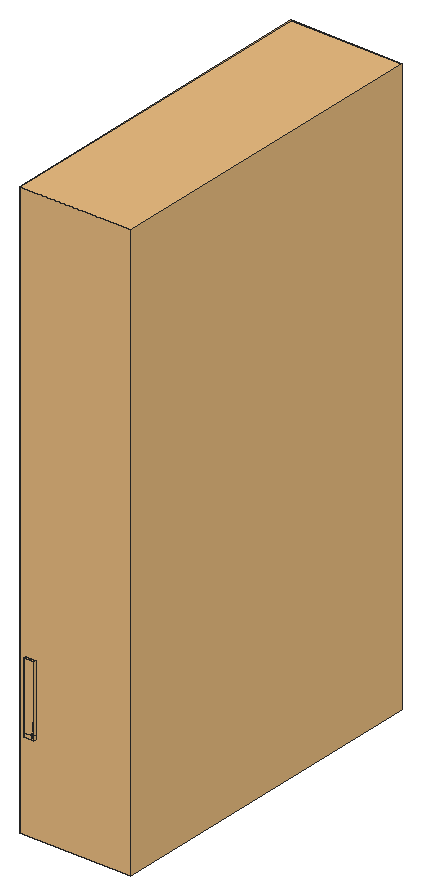
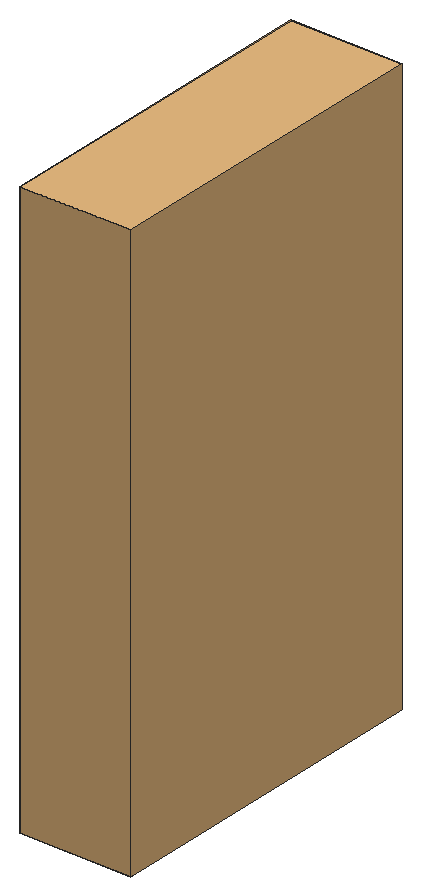
# SketchUp Ruby script. Lengths in inches.
U = 1.inch
M = Sketchup.active_model
def pt(a) = Geom::Point3d.new(a.map { |v| v * U })
def face(e, loops, mat)
  f = e.add_face(loops[0].map { |a| pt(a) })
  loops[1..].each { |l| e.add_face(l.map { |a| pt(a) }).erase! }
  f.material = f.back_material = mat if mat
  f
end
# faces: each face lists its corners as indices into pts; further lists are holes
def faces(e, pts, list, mat = nil) = list.each { |f| face(e, (f[0].is_a?(Array) ? f : [f]).map { |l| l.map { |i| pts[i] } }, mat) }
# xy, xz, yz: faces in a plane at the given z, y or x. An outline is a flat list of corners, or four numbers for a rectangle; further outlines are holes
def ring(l) = l.size == 4 ? [[l[0], l[1]], [l[2], l[1]], [l[2], l[3]], [l[0], l[3]]] : l.each_slice(2).to_a
def flat(e, list, mat, &to3) = list.each { |f| face(e, (f[0].is_a?(Array) ? f : [f]).map { |l| ring(l).map { |u, v| to3.(u, v) } }, mat) }
def xy(e, z, list, mat = nil) = flat(e, list, mat) { |x, y| [x, y, z] }
def xz(e, y, list, mat = nil) = flat(e, list, mat) { |x, z| [x, y, z] }
def yz(e, x, list, mat = nil) = flat(e, list, mat) { |y, z| [x, y, z] }
def lines(e, pts, list) = list.each { |a, b| e.add_line(pt(pts[a]), pt(pts[b])) }
# prism: a flat outline (further loops are holes) pulled along v
def prism(e, loops, v, mat = nil)
  f = face(e, loops, mat); d = Geom::Vector3d.new(v.map { |x| x * U })
  f.pushpull(f.normal.samedirection?(d) ? d.length : -d.length)
end
def box(e, o, s, mat = nil) = prism(e, [[o, [o[0] + s[0], o[1], o[2]], [o[0] + s[0], o[1] + s[1], o[2]], [o[0], o[1] + s[1], o[2]]]], [0, 0, s[2]], mat)
def at(x, y, z, deg = 0) = Geom::Transformation.translation(pt([x, y, z])) * Geom::Transformation.rotation(ORIGIN, Z_AXIS, deg.degrees)
def axes(o, x, y, z) = Geom::Transformation.new([*x, 0, *y, 0, *z, 0, *pt(o).to_a, 1])
def part(name) = M.definitions.add(name)
# library, detail: a bought-in or finely detailed component or shape, given as its bounding box
def library(name, o, s) = part(name).tap { |d| box(d.entities, o, s) }
def detail(e, o, s) = box(e.add_group.entities, o, s)
def put(e, d, t, mat = nil) = e.add_instance(d, t).tap { |i| i.material = mat if mat }
def group(e, t, mat = nil) = e.add_group.tap { |g| g.transformation = t; g.material = mat if mat }.entities
root = M.entities
M.materials.add("[Wood Cherry Original]").color = [152, 86, 42]
M.materials.add("green").color = [174, 139, 102]
M.materials.add("vio").color = [206, 114, 100]
c1 = library("3DGeom~135_Defintion",[-19.41,-483.5625,-70.5],[38.82,1000,141])
c2 = library("3DGeom~133_Defintion",[-19.91,-529.75,-72.32],[39.82,1000,144.37])
c3 = library("3DGeom~131_Defintion",[-19.41,-483.5625,-70.5],[38.82,1000,140.74])
c4 = part("3DGeom~134_Defintion")
p = [[-9.17,365.0625,-60.44],[-10.66,319.24,-60.24],[-9.24,319.23,-61.125],[-10.63,365.04,-59.53],[-12.34,365.04,-59.02],[-14.12,365.04,-58.98],
  [-14.05,319.22,-59.71],[-12.32,319.23,-59.75],[-8.56,277.89,-58.6875],[-8.45,241.12,-52.31],[-7.11,241.05,-53.13],[-9.93,277.92,-57.83],
  [-11.54,277.92,-57.36],[-13.22,277.89,-57.32],[-11.63,241.07,-51.81],[-10.01,241.13,-51.85],[-6.75,470.15,-49.68],[-9.84,415.33,-55.7],
  [-8.34,415.37,-56.63],[-8.29,470.08,-48.72],[-10.1,470.07,-48.1875],[-13.43,415.34,-55.13],[-11.6,415.32,-55.17],[-11.98,470.11,-48.14],
  [-4.1,211.43,-41.85],[-0.64,188.37,-23.41],[0.67,188.13,-24.11],[-5.42,211.6,-41.08],[-6.95,211.62,-40.63],[-8.53,211.47,-40.56],
  [-3.6875,188.18,-22.85],[-2.14,188.39,-22.97],[6.29,168.75,-2.9375],[10.49,151.32,19.02],[11.76,151.06,18.38],[6.29,168.75,-2.9375],
  [4.99,169.02,-2.29],[10.49,151.32,19.02],[3.51,169.05,-1.87],[2,168.82,-1.72],[7.55,151.14,19.55],[9.03,151.35,19.42],
  [-2.58,-7.65,9.24],[-5.6,-27.13,7.79],[-4.52,-27.2,7.15],[-3.69,-7.65,9.88],[-4.97,-7.58,10.22],[-6.28,-7.43,10.23],
  [-8.15,-27.06,8.11],[-6.85,-27.08,8.125],[-3.875,-43.53,12.625],[-2.45,-57.47,24.41],[-1.39,-57.67,23.87],[-4.94,-43.36,13.22],
  [-6.17,-43.32,13.55],[-7.45,-43.42,13.58],[-4.9,-57.59,24.83],[-3.66,-57.4375,24.75],[7.01,37.63,28.93],[0.5,14.23,18.1875],
  [1.64,14.26,17.55],[5.85,37.59,29.58],[4.53,37.68,29.94],[-2.125,14.51,18.57],[-0.8,14.3125,18.55],[3.18,37.89,29.97],
  [5.56,-294.46,30.13],[4.07,-328.71,26.72],[4.85,-328.71,26.23],[4.75,-294.51,30.64],[4.86,-362.1,26.86],[4.11,-362.08,27.33],
  [4.47,-395.52,30.27],[5.1875,-395.55,29.82],[3.8,-294.53,30.93],[2.8125,-294.51,30.96],[2.21,-328.71,27.03],[3.16,-328.71,27],
  [3.23,-362.08,27.6],[2.32,-362.08,27.63],[2.75,-395.51,30.56],[3.63,-395.5,30.53],[5.84,-429.05,35.11],[6.16,-462.54,43.14],
  [6.82,-462.6,42.73],[5.15,-429,35.54],[4.35,-428.98,35.79],[3.51,-428.99,35.8125],[4.58,-462.53,43.4],[5.39,-462.51,43.375],
  [16.05,132.58,36.39],[16.75,110.79,47.79],[17.95,110.68,47.08],[14.8125,132.8,37.06],[13.38,132.84,37.45],[11.91,132.69,37.51],
  [13.89,110.82,48.16],[15.34,110.84,48.16],[2.27,-71.39,38.47],[5.25,-86.23,54.01],[6.27,-86.4,53.46],[1.23,-71.18,39],
  [8.9,-222.87,50.33],[6.22,-258.8,39.57],[7.0625,-258.72,39.05],[0.04,-71.16,39.34],[-1.17,-71.33,39.4375],[2.89,-86.37,54.44],
  [4.09,-86.22,54.36],[8.03,-222.96,50.86],[7.01,-223,51.17],[5.95,-222.97,51.21],[4.22,-258.8,39.9],[5.24,-258.83,39.86],
  [16.42,86.25,47.3],[11.16,61.76,40.67],[12.34,61.78,40],[15.23,86.27,48],[13.86,86.35,48.37],[8.43,62.04,41.06],
  [9.8125,61.85,41.04],[12.44,86.47,48.36],[8.12,-496.2,52.69],[9.15,-529.77,65.34],[9.75,-529.85,64.98],[7.49,-496.125,53.08],
  [6.76,-496.1,53.3],[5.99,-496.12,53.32],[7.72,-529.76,65.58],[8.45,-529.74,65.55],[11.66,-156.24,69.3],[9.6875,-188.37,61.86],
  [10.59,-188.28,61.31],[10.73,-156.3,69.88],[9.64,-156.33,70.21],[8.51,-156.32,70.24],[7.54,-188.38,62.22],[8.64,-188.4,62.18],
  [9.71,-104.66,65.64],[8.72,-104.5625,66.23],[10.65,-127.92,72.15],[11.61,-127.92,71.55],[7.58,-104.56,66.57],[6.4,-104.66,66.625],
  [8.36,-127.96,72.52],[9.53,-127.93,72.49]]
faces(c4.entities,p,[[0,1,2],[0,3,1],[4,5,6],[4,6,7],[8,9,10],[8,11,9],[12,13,14],[12,14,15],
  [16,17,18],[16,19,17],[20,21,22],[20,23,21],[24,25,26],[24,27,25],[28,29,30],[28,30,31],
  [32,33,34],[35,36,37],[38,39,40],[38,40,41],[42,43,44],[42,45,43],[46,47,48],[46,48,49],
  [50,51,52],[50,53,51],[54,55,56],[54,56,57],[58,59,60],[58,61,59],[62,63,64],[62,65,63],
  [66,67,68],[66,69,67],[70,71,72],[70,72,73],[74,75,76],[74,76,77],[78,79,80],[78,80,81],
  [82,83,84],[82,85,83],[86,87,88],[86,88,89],[90,91,92],[90,93,91],[94,95,96],[94,96,97],
  [98,99,100],[98,101,99],[102,103,104],[105,106,107],[105,107,108],[102,109,103],[110,111,112],[110,112,113],
  [114,115,116],[114,117,115],[118,119,120],[118,121,119],[122,123,124],[122,125,123],[126,127,128],[126,128,129],
  [130,131,132],[130,133,131],[134,135,136],[134,136,137],[138,139,140],[138,140,141],[142,143,144],[142,144,145]],"green")
c5 = part("3DGeom~132_Defintion")
p = [[-9.01,311.27,-59.6],[-10.4,311.27,-58.74],[-9.6875,270.99,-56.39],[-8.34,270.95,-57.22],[-8.13,405.01,-55.22],[-10.37,355.9375,-58.05],
  [-8.94,355.96,-58.93],[-12.01,311.27,-58.26],[-13.69,311.26,-58.22],[-12.89,270.96,-55.89],[-11.25,270.99,-55.92],[-9.6,404.97,-54.31],
  [-11.31,404.95,-53.8],[-13.77,355.9375,-57.51],[-12.03,355.93,-57.55],[-13.1,404.98,-53.75],[-6.9375,235.04,-51.81],[-5.28,206.32,-40.06],
  [-3.99,206.16,-40.81],[-8.24,235.11,-51],[-9.76,235.11,-50.55],[-11.34,235.05,-50.51],[-8.32,206.19,-39.54],[-6.77,206.34,-39.62],
  [-4.28,516.18,-38.61],[-8.09,458.36,-47.51],[-6.58,458.42,-48.44],[-5.83,516.1,-37.65],[-7.64,516.08,-37.11],[-11.68,458.38,-46.9375],
  [-9.85,458.34,-46.98],[-9.53,516.13,-37.0625],[0.66,183.44,-23.51],[4.86,164.8,-2.23],[6.13,164.54,-2.87],[-0.625,183.67,-22.83],
  [-2.09,183.69,-22.4],[-3.59,183.49,-22.28],[1.95,164.61,-1.68],[3.42,164.83,-1.82],[-4.41,-26.52,6.97],[-4.82,-42.28,12.89],
  [-3.78,-42.44,12.31],[-5.46,-26.45,7.59],[-6.68,-26.4,7.92],[-7.95,-26.38,7.91],[-7.26,-42.34,13.24],[-6.02,-42.24,13.21],
  [1.59,13.9,17.11],[-3.6,-7.46,9.63],[-2.52,-7.46,9.01],[0.49,13.87,17.73],[-0.78,13.96,18.08],[-6.12,-7.25,9.97],
  [-4.84,-7.39,9.97],[-2.07,14.15,18.11],[11.47,147.29,17.92],[14.44,129.49,36.13],[15.65,129.27,35.48],[11.47,147.29,17.92],
  [10.22,147.54,18.54],[8.81,147.58,18.9375],[7.36,147.375,19.06],[11.62,129.38,36.57],[13.05,129.53,36.51],[-1.35,-56.24,23.27],
  [1.2,-69.4,38.03],[2.21,-69.6,37.51],[-2.38,-56.03,23.8],[-3.5625,-56,24.13],[-4.77,-56.16,24.21],[-1.15,-69.55,38.45],
  [0.04,-69.38,38.36],[4.73,-320.51,25.58],[3.97,-320.51,26.06],[4.01,-353.05,26.65],[4.74,-353.07,26.19],[3.08,-320.51,26.33],
  [2.15,-320.51,26.36],[2.26,-353.05,26.94],[3.15,-353.05,26.91],[12.03,60.24,39],[5.7,36.65,28.84],[6.83,36.6875,28.21],
  [10.88,60.22,39.65],[5.06,-385.68,29.08],[4.36,-385.65,29.52],[5.02,-418.3,34.66],[5.7,-418.34,34.23],[9.57,60.3,40.01],
  [3.1,36.95,29.23],[4.41,36.74,29.2],[8.22,60.49,40.03],[6.89,-252.26,38.07],[4.63,-287.17,29.875],[5.42,-287.12,29.38],
  [3.54,-385.64,29.77],[2.68,-385.64,29.79],[3.42,-418.29,34.92],[4.24,-418.28,34.89],[6.07,-252.34,38.58],[5.11,-252.37,38.87],
  [4.11,-252.34,38.9],[2.74,-287.17,30.1875],[3.71,-287.19,30.16],[6.65,-451.06,41.67],[7.3,-483.75,51.75],[7.92,-483.82,51.375],
  [6.01,-451,42.07],[5.26,-450.97,42.29],[4.47,-450.99,42.32],[5.84,-483.74,51.99],[6.59,-483.72,51.97],[17.5,107.92,45.9],
  [16.33,108.02,46.59],[14.85,84.12,46.8],[16.01,84.1,46.12],[14.96,108.07,46.96],[12.125,84.32,47.16],[13.51,84.19,47.16],
  [13.54,108.06,46.96],[10.32,-183.58,59.78],[7.83,-217.4,49.6],[8.67,-217.31,49.07],[9.44,-183.67,60.32],[8.42,-183.7,60.63],
  [7.35,-183.68,60.66],[5.8,-217.4,49.93],[6.83,-217.43,49.89],[6.11,-84.25,52.125],[8.51,-101.95,64.58],[9.47,-102.05,64],
  [5.12,-84.08,52.67],[3.99,-84.07,53],[2.82,-84.22,53.08],[6.24,-102.05,64.96],[7.39,-101.95,64.91],[11.32,-124.73,69.76],
  [10.46,-152.4,68.13],[11.37,-152.34,67.57],[10.39,-124.73,70.35],[9.3,-124.74,70.69],[8.15,-124.76,70.71],[8.29,-152.42,68.49],
  [9.4,-152.43,68.46]]
faces(c5.entities,p,[[0,1,2],[0,2,3],[4,5,6],[7,8,9],[7,9,10],[4,11,5],[12,13,14],[12,15,13],
  [16,17,18],[16,19,17],[20,21,22],[20,22,23],[24,25,26],[24,27,25],[28,29,30],[28,31,29],
  [32,33,34],[32,35,33],[36,37,38],[36,38,39],[40,41,42],[40,43,41],[44,45,46],[44,46,47],
  [48,49,50],[48,51,49],[52,53,54],[52,55,53],[56,57,58],[59,60,57],[61,62,63],[61,63,64],
  [65,66,67],[65,68,66],[69,70,71],[69,71,72],[73,74,75],[73,75,76],[77,78,79],[77,79,80],
  [81,82,83],[81,84,82],[85,86,87],[85,87,88],[89,90,91],[89,92,90],[93,94,95],[96,97,98],
  [96,98,99],[93,100,94],[101,102,103],[101,103,104],[105,106,107],[105,108,106],[109,110,111],[109,111,112],
  [113,114,115],[113,115,116],[117,118,119],[117,120,118],[121,122,123],[121,124,122],[125,126,127],[125,127,128],
  [129,130,131],[129,132,130],[133,134,135],[133,135,136],[137,138,139],[137,140,138],[141,142,143],[141,143,144]],"green")
c6 = part("3DGeom~130_Defintion")
p = [[-10.63,365.1,-59.54],[-12.32,319.28,-59.76],[-10.66,319.28,-60.25],[-12.34,365.09,-59.03],[-9.9375,277.96,-57.84],[-11.54,277.96,-57.36],
  [-10.01,241.16,-51.85],[-8.45,241.16,-52.32],[-8.3,470.15,-48.73],[-11.6,415.375,-55.18],[-9.85,415.39,-55.7],[-10.1,470.14,-48.19],
  [-5.42,211.63,-41.09],[-6.95,211.65,-40.64],[-2.14,188.42,-22.97],[-0.64,188.4,-23.41],[4.99,169.04,-2.29],[9.03,151.375,19.43],
  [10.49,151.34,19.02],[3.51,169.07,-1.87],[-3.69,-7.65,9.88],[-6.85,-27.08,8.125],[-5.6,-27.13,7.79],[-4.97,-7.58,10.23],
  [-4.94,-43.37,13.22],[-3.66,-57.45,24.75],[-2.45,-57.48,24.42],[-6.18,-43.33,13.55],[5.85,37.6,29.58],[-0.8,14.32,18.55],
  [0.5,14.23,18.19],[4.53,37.6875,29.95],[4.75,-294.56,30.64],[3.16,-328.76,27.01],[4.07,-328.76,26.73],[3.8,-294.58,30.93],
  [4.11,-362.14,27.34],[3.23,-362.13,27.61],[3.63,-395.56,30.53],[4.47,-395.57,30.28],[5.15,-429.0625,35.55],[4.35,-429.04,35.79],
  [5.39,-462.58,43.38],[6.16,-462.6,43.15],[14.8125,132.82,37.06],[15.35,110.85,48.17],[16.75,110.8,47.79],[13.39,132.86,37.45],
  [1.23,-71.19,39],[0.04,-71.17,39.34],[4.09,-86.23,54.36],[5.25,-86.24,54.02],[8.03,-222.99,50.87],[5.24,-258.86,39.87],
  [6.22,-258.83,39.57],[7.01,-223.03,51.18],[15.23,86.29,48],[9.81,61.86,41.04],[11.16,61.77,40.67],[13.86,86.36,48.375],
  [7.49,-496.2,53.08],[6.76,-496.17,53.3],[8.45,-529.82,65.5625],[9.15,-529.85,65.35],[10.73,-156.33,69.89],[8.64,-188.43,62.1875],
  [9.6875,-188.39,61.87],[9.64,-156.35,70.22],[8.73,-104.58,66.24],[7.58,-104.57,66.58],[9.53,-127.95,72.5],[10.66,-127.9375,72.16]]
faces(c6.entities,p,[[0,1,2],[0,3,1],[4,5,6],[4,6,7],[8,9,10],[8,11,9],[12,13,14],[12,14,15],
  [16,17,18],[16,19,17],[20,21,22],[20,23,21],[24,25,26],[24,27,25],[28,29,30],[28,31,29],
  [32,33,34],[32,35,33],[36,37,38],[36,38,39],[40,41,42],[40,42,43],[44,45,46],[44,47,45],
  [48,49,50],[48,50,51],[52,53,54],[52,55,53],[56,57,58],[56,59,57],[60,61,62],[60,62,63],
  [64,65,66],[64,67,65],[68,69,70],[68,70,71]],"green")
c7 = part("3DGeom~129_Defintion")
p = [[-10.4,311.32,-58.75],[-12.01,311.32,-58.27],[-11.25,271.03,-55.93],[-9.6875,271.03,-56.4],[-9.6,405.03,-54.31],[-12.03,355.98,-57.5625],
  [-10.37,355.99,-58.06],[-11.3125,405.02,-53.8],[-8.24,235.14,-51.01],[-9.76,235.15,-50.5625],[-6.78,206.37,-39.62],[-5.28,206.35,-40.0625],
  [-5.83,516.18,-37.66],[-9.85,458.41,-46.99],[-8.09,458.42,-47.52],[-7.64,516.16,-37.12],[-0.625,183.7,-22.83],[3.42,164.86,-1.82],
  [4.87,164.83,-2.23],[-2.09,183.72,-22.4],[-5.46,-26.46,7.59],[-6.68,-26.41,7.92],[-6.02,-42.25,13.22],[-4.82,-42.29,12.89],
  [0.49,13.875,17.74],[-4.84,-7.39,9.97],[-3.6,-7.46,9.63],[-0.78,13.96,18.09],[10.23,147.57,18.54],[8.81,147.6,18.94],
  [13.05,129.54,36.52],[14.44,129.5,36.14],[-2.39,-56.04,23.81],[-3.56,-56.01,24.13],[0.04,-69.39,38.36],[1.2,-69.42,38.03],
  [3.97,-320.56,26.0625],[3.08,-320.5625,26.33],[3.15,-353.1,26.92],[4.01,-353.11,26.65],[10.88,60.23,39.66],[4.41,36.75,29.2],
  [5.7,36.66,28.85],[9.57,60.3125,40.02],[4.36,-385.71,29.52],[4.24,-418.34,34.9],[5.02,-418.36,34.66],[3.54,-385.69,29.77],
  [6.07,-252.38,38.58],[3.71,-287.23,30.16],[4.63,-287.21,29.88],[5.11,-252.41,38.875],[6.01,-451.07,42.07],[5.26,-451.04,42.3],
  [6.59,-483.8,51.97],[7.31,-483.82,51.76],[16.33,108.04,46.6],[13.51,84.21,47.17],[14.85,84.13,46.81],[14.96,108.09,46.97],
  [9.45,-183.7,60.33],[6.84,-217.47,49.9],[7.83,-217.43,49.6],[8.42,-183.73,60.64],[5.12,-84.09,52.67],[3.99,-84.08,53.01],
  [7.39,-101.97,64.92],[8.51,-101.97,64.59],[10.39,-124.75,70.36],[9.4,-152.46,68.47],[10.46,-152.43,68.15],[9.3,-124.76,70.7]]
faces(c7.entities,p,[[0,1,2],[0,2,3],[4,5,6],[4,7,5],[8,9,10],[8,10,11],[12,13,14],[12,15,13],
  [16,17,18],[16,19,17],[20,21,22],[20,22,23],[24,25,26],[24,27,25],[28,29,30],[28,30,31],
  [32,33,34],[32,34,35],[36,37,38],[36,38,39],[40,41,42],[40,43,41],[44,45,46],[44,47,45],
  [48,49,50],[48,51,49],[52,53,54],[52,54,55],[56,57,58],[56,59,57],[60,61,62],[60,63,61],
  [64,65,66],[64,66,67],[68,69,70],[68,71,69]],"green")
c8 = part("3DGeom~212_Defintion")
p = [[-253.96,-102.22,-418.25],[-4.58,-88.53,-492.98],[51.95,-256.53,-399.89],[278.67,-148.1,-381.875],[51.95,-256.53,-399.89],[246.04,-51.11,-435.625],
  [-251.19,119.16,-413.67],[-253.96,-102.22,-418.25],[-251.19,119.16,-413.67],[-2.17,103.2,-489.02],[247.42,59.58,-433.34],[58.52,267.27,-389.07],
  [-181.11,308.61,-298.26],[-251.19,119.16,-413.67],[-181.11,308.61,-298.26],[278.67,-148.1,-381.875],[246.04,-51.11,-435.625],[430.72,0,-261.54],
  [430.72,0,-261.54],[247.42,59.58,-433.34],[282.46,154.31,-375.63],[282.46,154.31,-375.63],[-435.3,-88.53,-231.44],[-253.96,-102.22,-418.25],
  [-188.69,-296.21,-310.75],[-253.96,-102.22,-418.25],[51.95,-256.53,-399.89],[-188.69,-296.21,-310.75],[-432.9,103.2,-227.48],[-251.19,119.16,-413.67],
  [-372.21,267.26,-127.53],[-181.11,308.61,-298.26],[-188.69,-296.21,-310.75],[51.95,-256.53,-399.89],[152.27,-355.79,-234.68],[51.95,-256.53,-399.89],
  [336.59,-205.41,-286.49],[152.27,-355.79,-234.68],[51.95,-256.53,-399.89],[336.59,-205.41,-286.49],[161.24,359.72,-219.91],[-62.5,415.37,-102.93],
  [58.52,267.27,-389.07],[-181.11,308.61,-298.26],[161.24,359.72,-219.91],[58.52,267.27,-389.07],[336.59,-205.41,-286.49],[278.67,-148.1,-381.875],
  [282.46,154.31,-375.63],[341.77,207.68,-277.97],[161.24,359.72,-219.91],[341.77,207.68,-277.97],[-378.77,-256.53,-138.34],[-72.86,-410.83,-119.99],
  [-188.69,-296.21,-310.75],[-378.77,-256.53,-138.34],[-269.49,359.72,41.63],[-181.11,308.61,-298.26],[-372.21,267.26,-127.53],[-269.49,359.72,41.63],
  [-181.11,308.61,-298.26],[336.59,-205.41,-286.49],[404.27,-207.68,-175.04],[404.27,-207.68,-175.04],[336.59,-205.41,-286.49],[341.77,207.68,-277.97],
  [409.45,205.41,-166.51],[278.46,355.79,-26.86],[409.45,205.41,-166.51],[341.77,207.68,-277.97],[341.77,207.68,-277.97],[463.57,-154.31,-77.37],
  [498.61,-59.58,-19.66],[500,51.11,-17.38],[409.45,205.41,-166.51],[467.36,148.11,-71.13],[269.49,-359.72,-41.63],[404.27,-207.68,-175.04],
  [-500,-51.11,17.38],[-498.61,59.58,19.66],[-463.57,154.3,77.37],[72.86,410.83,119.98],[269.49,-359.72,-41.63],[378.77,256.53,138.34],
  [409.45,205.41,-166.51],[378.77,256.53,138.34],[409.45,205.41,-166.51],[278.46,355.79,-26.86],[-378.77,-256.53,-138.34],[-278.46,-355.79,26.86],
  [-467.36,-148.11,71.13],[-278.46,-355.79,26.86],[-404.27,207.68,175.04],[-269.49,359.72,41.63],[62.5,-415.37,102.93],[-152.27,355.79,234.68],
  [-269.49,359.72,41.63],[269.49,-359.72,-41.63],[372.21,-267.27,127.53],[435.3,88.53,231.44],[378.77,256.53,138.34],[372.21,-267.27,127.53],
  [188.69,296.21,310.75],[378.77,256.53,138.34],[432.9,-103.2,227.48],[-430.72,0,261.54],[-161.24,-359.72,219.91],[-409.45,-205.41,166.51],
  [-161.24,-359.72,219.91],[-278.46,-355.79,26.86],[-409.45,-205.41,166.51],[-336.59,205.41,286.49],[-269.49,359.72,41.63],[-404.27,207.68,175.04],
  [-336.59,205.41,286.49],[-269.49,359.72,41.63],[-161.24,-359.72,219.91],[181.11,-308.61,298.26],[372.21,-267.27,127.53],[181.11,-308.61,298.26],
  [-51.95,256.53,399.89],[-51.95,256.53,399.89],[181.11,-308.61,298.26],[253.96,102.22,418.25],[378.77,256.53,138.34],[253.96,102.22,418.25],
  [378.77,256.53,138.34],[188.69,296.21,310.75],[-409.45,-205.41,166.51],[-161.24,-359.72,219.91],[-341.77,-207.68,277.97],[-341.77,-207.68,277.97],
  [-336.59,205.41,286.49],[-341.77,-207.68,277.97],[-161.24,-359.72,219.91],[-58.52,-267.27,389.07],[-161.24,-359.72,219.91],[181.11,-308.61,298.26],
  [-58.52,-267.27,389.07],[181.11,-308.61,298.26],[251.1875,-119.16,413.67],[251.1875,-119.16,413.67],[251.1875,-119.16,413.67],[253.96,102.22,418.25],
  [-278.67,148.1,381.875],[-152.27,355.79,234.68],[-336.59,205.41,286.49],[-278.67,148.1,381.875],[-51.95,256.53,399.89],[-152.27,355.79,234.68],
  [-282.46,-154.31,375.63],[-247.42,-59.58,433.34],[-247.42,-59.58,433.34],[-246.04,51.11,435.625],[-430.72,0,261.54],[-278.67,148.1,381.875],
  [-246.04,51.11,435.625],[-341.77,-207.68,277.97],[-282.46,-154.31,375.63],[181.11,-308.61,298.26],[251.1875,-119.16,413.67],[4.58,88.53,492.98],
  [188.69,296.21,310.75],[253.96,102.22,418.25],[188.69,296.21,310.75],[-282.46,-154.31,375.63],[2.17,-103.2,489.02],[-282.46,-154.31,375.63],
  [-247.42,-59.58,433.34],[-246.04,51.11,435.625],[-278.67,148.1,381.875],[-246.04,51.11,435.625],[-247.42,-59.58,433.34],[-247.42,-59.58,433.34],
  [-246.04,51.11,435.625]]
faces(c8.entities,p,[[0,1,2],[1,3,4],[1,5,3],[6,1,7],[8,9,1],[9,5,1],[9,10,5],[11,10,9],
  [12,9,13],[14,11,9],[15,16,17],[5,10,18],[19,20,17],[11,21,10],[22,23,24],[25,26,27],
  [28,23,22],[28,29,23],[30,29,28],[30,31,29],[32,33,34],[35,36,37],[38,3,39],[40,21,11],
  [41,42,43],[41,44,45],[46,47,17],[48,49,17],[50,51,21],[52,32,53],[32,34,53],[22,54,55],
  [56,57,58],[59,41,60],[34,61,62],[63,64,17],[65,66,17],[67,68,69],[67,70,44],[71,63,17],
  [72,71,17],[73,72,17],[74,75,17],[75,73,17],[53,34,76],[34,77,76],[78,22,55],[79,22,78],
  [79,28,22],[80,28,79],[80,30,28],[81,67,44],[81,44,41],[82,63,71],[83,75,84],[85,86,87],
  [88,53,89],[90,55,91],[78,55,90],[92,30,80],[92,93,30],[89,53,94],[53,76,94],[95,41,96],
  [95,81,41],[97,71,98],[98,71,72],[99,73,75],[99,75,100],[94,76,101],[102,103,67],[102,67,81],
  [98,72,104],[104,72,73],[104,73,99],[78,90,105],[79,78,105],[80,79,105],[89,94,106],[107,89,108],
  [90,109,110],[111,112,113],[114,95,115],[90,110,105],[92,80,105],[116,94,117],[94,118,119],[120,81,95],
  [121,102,81],[122,98,104],[123,99,124],[125,126,127],[128,129,130],[110,131,105],[132,92,105],[133,134,135],
  [136,137,138],[139,104,140],[141,104,99],[142,99,143],[144,145,146],[147,148,149],[131,150,105],[150,151,105],
  [152,153,154],[155,132,105],[156,155,105],[157,135,158],[135,159,160],[161,162,148],[161,163,164],[165,135,166],
  [167,166,168],[169,148,170],[135,160,166],[171,161,148],[166,160,163],[166,163,161],[172,166,161],[173,161,174]],"vio")
c9 = library("3DGeom~146_Defintion",[-500,-464.96,-145.56],[1000,929.92,291.12])
c10 = part("3DGeom~147_Defintion")
p = [[447.11,-464.11,-119.78],[466.43,-447.31,-145.56],[454.24,-459.97,-82.98],[466.43,-447.31,-145.56],[447.11,-464.11,-119.78],[454.17,-457.65,-136.37],
  [454.24,-459.97,-82.98],[466.43,-447.31,-145.56],[480.68,-439.04,-71.95],[466.43,-447.31,-145.56],[480.59,-435.86,-144.88],[492.87,-426.375,-134.53],
  [500,-422.24,-97.72],[466.43,-447.31,-145.56],[492.87,-426.375,-134.53],[480.68,-439.04,-71.95],[466.43,-447.31,-145.56],[492.87,-426.375,-134.53],
  [499.98,-421.39,-117.27],[447.11,-464.11,-119.78],[454.24,-459.97,-82.98],[447.13,-464.96,-100.24],[480.68,-439.04,-71.95],[492.9375,-428.7,-81.14],
  [454.24,-459.97,-82.98],[480.68,-439.04,-71.95],[466.52,-450.48,-72.62],[-486.65,450.01,82.87],[-454.24,464.96,91.16],[-470.88,459.85,82.8125],
  [-486.65,450.01,82.87],[-494.01,420.39,122.7],[-480.9375,419.38,137.21],[-486.65,450.01,82.87],[-480.9375,419.38,137.21],[-464.29,424.49,145.56],
  [-486.65,450.01,82.87],[-500,427.23,105.9],[-494.01,420.39,122.7],[-486.65,450.01,82.87],[-464.29,424.49,145.56],[-448.53,434.33,145.5],
  [-486.65,450.01,82.87],[-497.31,438.07,91.32],[-500,427.23,105.9],[-486.65,450.01,82.87],[-448.53,434.33,145.5],[-437.87,446.27,137.04],
  [-486.65,450.01,82.87],[-437.87,446.27,137.04],[-435.17,457.12,122.47],[-486.65,450.01,82.87],[-441.17,463.96,105.67],[-454.24,464.96,91.16],
  [-486.65,450.01,82.87],[-435.17,457.12,122.47]]
faces(c10.entities,p,[[0,1,2],[3,4,5],[6,7,8],[9,10,11],[12,13,14],[15,16,12],[12,17,18],[19,20,21],
  [22,12,23],[24,25,26],[27,28,29],[30,31,32],[33,34,35],[36,37,38],[39,40,41],[42,43,44],
  [45,46,47],[48,49,50],[51,52,53],[54,55,52]],"green")
c11 = part("3DGeom~235_Defintion")
p = [[111.34,-218.38,-429.9],[-247.29,-210.43,-375.22],[-78.46,-72.24,-500],[275.78,-41.25,-430.1],[-393.46,-67.1,-319.9],[-393.46,-67.1,-319.9],
  [-247.23,93.26,-436.12],[111.4,85.3125,-490.8],[366.3125,146.93,-315.04],[-34.76,228.64,-435.48],[271.41,220,-350.09],[366.3125,146.93,-315.04],
  [271.41,220,-350.09],[-247.23,93.26,-436.12],[-393.46,-67.1,-319.9],[-482.25,54.59,-163.38],[-247.23,93.26,-436.12],[-349.76,233.77,-255.38],
  [-349.76,233.77,-255.38],[271.41,220,-350.09],[187.03,302.75,-318.15],[-349.76,233.77,-255.38],[-123.56,350.33,-278.96],[187.03,302.75,-318.15],
  [-123.56,350.33,-278.96],[414.31,-117.14,-269.63],[446.3,103.11,-222.4],[414.31,-117.14,-269.63],[275.78,-41.25,-430.1],[275.78,-41.25,-430.1],
  [366.3125,146.93,-315.04],[-82.92,-337,-314.52],[271.31,-306.01,-244.62],[-82.92,-337,-314.52],[111.34,-218.38,-429.9],[414.31,-117.14,-269.63],
  [271.31,-306.01,-244.62],[-82.92,-337,-314.52],[-349.87,-292.24,-149.91],[-247.29,-210.43,-375.22],[-247.29,-210.43,-375.22],[-349.87,-292.24,-149.91],
  [-434.26,-209.49,-117.97],[-247.29,-210.43,-375.22],[271.41,220,-350.09],[358.7,295.74,-115.58],[187.03,302.75,-318.15],[-485.52,-139.23,-27.6],
  [187.03,302.75,-318.15],[135.76,373.01,-227.78],[358.7,295.74,-115.58],[187.03,302.75,-318.15],[-123.56,350.33,-278.96],[135.76,373.01,-227.78],
  [55.61,-412.89,-154.05],[-254.97,-365.3125,-114.86],[-82.92,-337,-314.52],[271.31,-306.01,-244.62],[-82.92,-337,-314.52],[-82.92,-337,-314.52],
  [-349.87,-292.24,-149.91],[-123.56,350.33,-278.96],[-349.76,233.77,-255.38],[-358.58,311.65,-6.22],[-131.1875,417.76,-63.17],[489.89,-122.02,-52.4],
  [271.31,-306.01,-244.62],[489.93,100.3,-96.98],[-349.76,233.77,-255.38],[-489.89,122.02,52.4],[-349.76,233.77,-255.38],[-358.58,311.65,-6.22],
  [358.58,-311.65,6.22],[271.31,-306.01,-244.62],[358.58,-311.65,6.22],[271.31,-306.01,-244.62],[131.35,411.94,-103.2],[358.7,295.74,-115.58],
  [-489.93,-100.3,96.98],[131.1875,-417.76,63.17],[-174.99,-409.125,-22.22],[358.58,-311.65,6.22],[-254.97,-365.3125,-114.86],[-358.7,-295.74,115.58],
  [-358.7,-295.74,115.58],[-358.7,-295.74,115.58],[485.52,139.23,27.6],[434.26,209.49,117.97],[349.87,292.24,149.91],[254.97,365.3125,114.86],
  [174.99,409.125,22.22],[358.7,295.74,-115.58],[254.97,365.3125,114.86],[358.7,295.74,-115.58],[-358.7,-295.74,115.58],[-55.61,412.89,154.05],
  [-271.31,306.01,244.62],[482.25,-54.59,163.38],[-358.7,-295.74,115.58],[-131.35,-411.94,103.2],[-358.58,311.65,-6.22],[-414.31,117.14,269.63],
  [-358.58,311.65,-6.22],[-414.31,117.14,269.63],[-271.31,306.01,244.62],[349.76,-233.77,255.39],[358.58,-311.65,6.22],[349.76,-233.77,255.39],
  [82.92,337,314.52],[254.97,365.3125,114.86],[-446.3,-103.11,222.4],[-414.31,117.14,269.63],[123.56,-350.33,278.96],[349.76,-233.77,255.39],
  [-358.7,-295.74,115.58],[-135.76,-373.01,227.78],[254.97,365.3125,114.86],[247.29,210.43,375.22],[254.97,365.3125,114.86],[247.29,210.43,375.22],
  [349.87,292.24,149.91],[-187.03,-302.75,318.15],[-187.03,-302.75,318.15],[-271.41,-220,350.09],[-358.7,-295.74,115.58],[-366.31,-146.93,315.04],
  [-358.7,-295.74,115.58],[-271.41,-220,350.09],[-366.31,-146.93,315.04],[-358.7,-295.74,115.58],[393.46,67.1,319.9],[247.29,210.43,375.22],
  [-111.34,218.38,429.9],[-111.34,218.38,429.9],[-414.31,117.14,269.63],[-366.31,-146.93,315.04],[34.76,-228.64,435.48],[-187.03,-302.75,318.15],
  [-135.76,-373.01,227.78],[-135.76,-373.01,227.78],[123.56,-350.33,278.96],[-271.31,306.01,244.62],[-414.31,117.14,269.63],[-275.78,41.25,430.1],
  [-111.34,218.38,429.9],[247.23,-93.26,436.12],[123.56,-350.33,278.96],[349.76,-233.77,255.39],[247.23,-93.26,436.12],[-414.31,117.14,269.63],
  [-366.31,-146.93,315.04],[-275.78,41.25,430.1],[247.23,-93.26,436.12],[123.56,-350.33,278.96],[82.92,337,314.52],[78.46,72.24,500],
  [82.92,337,314.52],[247.29,210.43,375.22],[-366.31,-146.93,315.04],[-271.41,-220,350.09],[-111.4,-85.3125,490.8],[247.29,210.43,375.22],
  [247.23,-93.26,436.12],[393.46,67.1,319.9],[247.29,210.43,375.22],[247.23,-93.26,436.12],[247.23,-93.26,436.12]]
faces(c11.entities,p,[[0,1,2],[3,0,2],[2,1,4],[2,5,6],[7,2,6],[3,2,7],[8,3,7],[7,6,9],
  [10,7,9],[11,7,12],[13,14,15],[16,15,17],[9,6,18],[19,9,20],[9,21,22],[23,9,24],
  [25,0,3],[26,27,28],[26,29,30],[0,31,1],[32,33,34],[35,36,0],[37,38,39],[40,41,42],
  [43,42,14],[30,44,45],[44,46,45],[14,42,47],[14,47,15],[48,49,50],[51,52,53],[26,30,45],
  [54,55,56],[57,54,58],[59,55,60],[61,62,63],[61,63,64],[49,61,64],[65,66,27],[67,65,27],
  [67,27,26],[68,15,69],[70,69,71],[72,54,73],[65,74,75],[49,76,77],[49,64,76],[67,26,45],
  [15,47,78],[15,78,69],[79,80,54],[81,79,54],[54,80,55],[41,82,83],[42,41,84],[47,42,85],
  [86,67,45],[87,86,45],[88,87,45],[89,88,45],[76,90,91],[90,92,93],[55,80,94],[76,95,90],
  [76,64,95],[86,65,67],[64,63,96],[64,96,95],[97,74,65],[86,97,65],[78,47,98],[79,99,80],
  [80,99,94],[100,69,101],[102,103,104],[105,79,106],[97,107,74],[90,95,108],[90,108,109],[87,97,86],
  [69,78,110],[69,110,111],[112,99,79],[113,112,79],[110,78,114],[99,115,94],[112,115,99],[116,108,117],
  [118,119,120],[115,121,94],[122,123,124],[125,110,126],[127,128,129],[87,130,97],[88,130,87],[88,131,130],
  [95,96,132],[95,133,108],[130,107,97],[134,110,135],[136,137,138],[136,139,140],[141,142,143],[141,143,144],
  [145,146,147],[130,148,107],[149,150,151],[152,136,153],[154,144,155],[156,155,157],[143,158,159],[160,159,137],
  [160,137,136],[161,162,163],[143,159,160],[164,155,165],[144,143,160],[144,160,155],[155,160,136],[155,136,166]],"vio")
c12 = library("Group\#39",[0,-13.41,-10],[36,16.82,88])
c13 = library("flowers vase",[13.94,34.08,0],[79.78,27.28,49.07])
put(root,c1,axes([13.77,135.02,35.07],[0,0.0104,0],[0,0,-0.0104],[-0.0104,0,0]),"green")
put(root,c2,axes([13.77,135.02,35.07],[0,0.01014,0],[0,0,-0.01014],[-0.01014,0,0]),"green")
put(root,c3,axes([13.77,135.02,35.07],[0,0.0104,0],[0,0,-0.0104],[-0.0104,0,0]),"green")
put(root,c4,axes([13.77,135.02,35.07],[0,0.01011,0],[0,0,-0.01011],[-0.01011,0,0]),"green")
put(root,c5,axes([13.77,135.02,35.07],[0,0.01037,0],[0,0,-0.01037],[-0.01037,0,0]),"green")
put(root,c6,axes([13.77,135.02,35.07],[0,0.01011,0],[0,0,-0.01011],[-0.01011,0,0]),"green")
put(root,c7,axes([13.77,135.02,35.07],[0,0.01037,0],[0,0,-0.01037],[-0.01037,0,0]),"green")
g1 = group(root,at(15.3125,134.49,26.21))
put(g1,c8,axes([-2.15,0.57,6.42],[0,0.00039,0],[0,0,-0.00039],[-0.00039,0,0]),"vio")
g2 = group(root,at(15.3125,134.49,26.21))
put(g2,c9,axes([-1.92,0.83,7.88],[0,0.00039,0],[0,0,-0.00039],[-0.00039,0,0]),"green")
put(g2,c10,axes([-1.92,0.83,7.88],[0,0.00039,0],[0,0,-0.00039],[-0.00039,0,0]),"green")
g3 = group(root,at(15.3125,134.49,26.21))
put(g3,c11,axes([-1.87,1.05,8.08],[0,0.00038,0],[0,0,-0.00038],[-0.00038,0,0]),"vio")
put(root,c12,axes([6.5,146.52,18],[0,1.43,0],[-1,0,0],[0,0,1]),"[Wood Cherry Original]")
put(root,c13,axes([0.77,193.625,19],[0,-0.24,0],[0.24,0,0],[0,0,0.24]))
